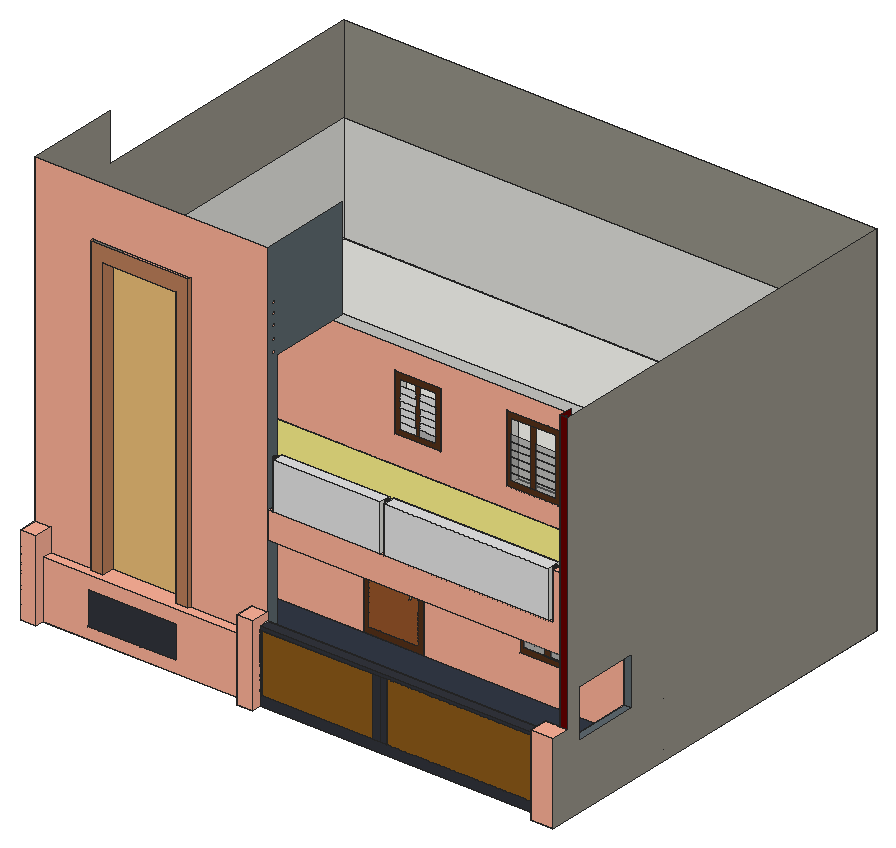
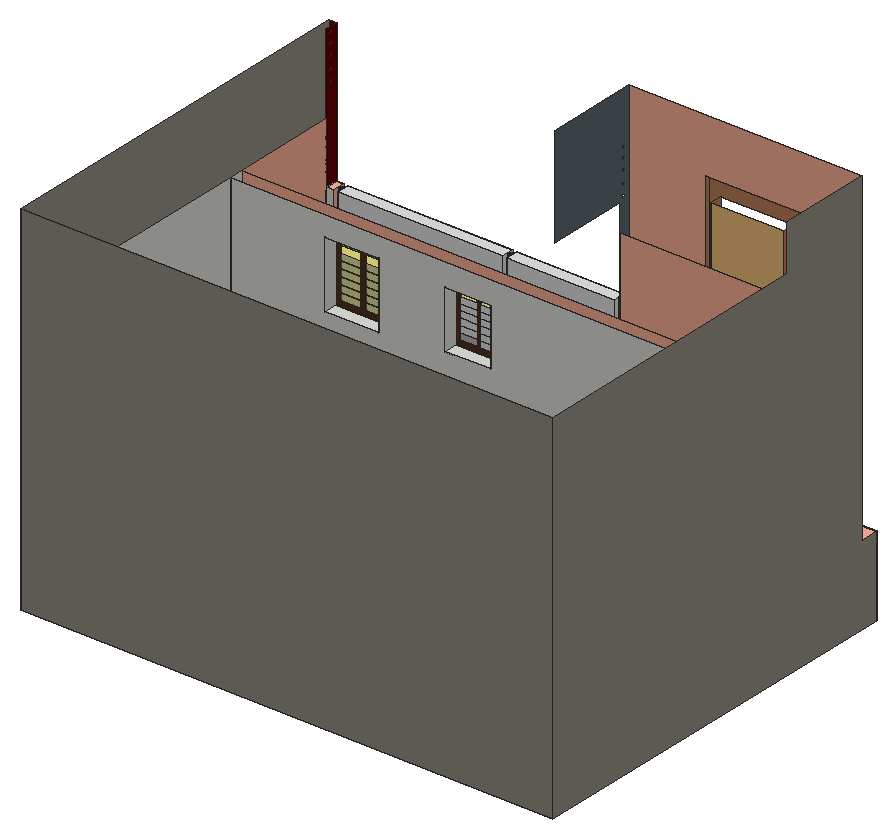
# SketchUp Ruby script. Lengths in inches.
U = 1.inch
M = Sketchup.active_model
def pt(a) = Geom::Point3d.new(a.map { |v| v * U })
def face(e, loops, mat)
  f = e.add_face(loops[0].map { |a| pt(a) })
  loops[1..].each { |l| e.add_face(l.map { |a| pt(a) }).erase! }
  f.material = f.back_material = mat if mat
  f
end
# faces: each face lists its corners as indices into pts; further lists are holes
def faces(e, pts, list, mat = nil) = list.each { |f| face(e, (f[0].is_a?(Array) ? f : [f]).map { |l| l.map { |i| pts[i] } }, mat) }
# xy, xz, yz: faces in a plane at the given z, y or x. An outline is a flat list of corners, or four numbers for a rectangle; further outlines are holes
def ring(l) = l.size == 4 ? [[l[0], l[1]], [l[2], l[1]], [l[2], l[3]], [l[0], l[3]]] : l.each_slice(2).to_a
def flat(e, list, mat, &to3) = list.each { |f| face(e, (f[0].is_a?(Array) ? f : [f]).map { |l| ring(l).map { |u, v| to3.(u, v) } }, mat) }
def xy(e, z, list, mat = nil) = flat(e, list, mat) { |x, y| [x, y, z] }
def xz(e, y, list, mat = nil) = flat(e, list, mat) { |x, z| [x, y, z] }
def yz(e, x, list, mat = nil) = flat(e, list, mat) { |y, z| [x, y, z] }
def lines(e, pts, list) = list.each { |a, b| e.add_line(pt(pts[a]), pt(pts[b])) }
# prism: a flat outline (further loops are holes) pulled along v
def prism(e, loops, v, mat = nil)
  f = face(e, loops, mat); d = Geom::Vector3d.new(v.map { |x| x * U })
  f.pushpull(f.normal.samedirection?(d) ? d.length : -d.length)
end
def box(e, o, s, mat = nil) = prism(e, [[o, [o[0] + s[0], o[1], o[2]], [o[0] + s[0], o[1] + s[1], o[2]], [o[0], o[1] + s[1], o[2]]]], [0, 0, s[2]], mat)
def at(x, y, z, deg = 0) = Geom::Transformation.translation(pt([x, y, z])) * Geom::Transformation.rotation(ORIGIN, Z_AXIS, deg.degrees)
def axes(o, x, y, z) = Geom::Transformation.new([*x, 0, *y, 0, *z, 0, *pt(o).to_a, 1])
def part(name) = M.definitions.add(name)
# library, detail: a bought-in or finely detailed component or shape, given as its bounding box
def library(name, o, s) = part(name).tap { |d| box(d.entities, o, s) }
def detail(e, o, s) = box(e.add_group.entities, o, s)
def put(e, d, t, mat = nil) = e.add_instance(d, t).tap { |i| i.material = mat if mat }
def group(e, t, mat = nil) = e.add_group.tap { |g| g.transformation = t; g.material = mat if mat }.entities
root = M.entities
M.materials.add("[Blinds Weave]").color = [141, 91, 25]
M.materials.add("[Carpet Diamond Yellow]").color = [226, 217, 124]
M.materials.add("[Color A08]").color = [102, 0, 0]
M.materials.add("[Color B02]").color = [255, 178, 153]
M.materials.add("[Formica Graystone]").color = [149, 146, 135]
M.materials.add("[Formica Laminate Dark]").color = [50, 53, 60]
M.materials.add("[Formica Speckled Grey]").color = [94, 105, 111]
M.materials.add("[Mirror 01]").color = [185, 185, 185]
M.materials.add("[Mirror 02]").color = [229, 229, 229]
M.materials.add("[Suede Blue]").color = [50, 57, 70]
M.materials.add("[Translucent Glass Gray]").color = [128, 128, 128]
M.materials["[Translucent Glass Gray]"].alpha = 0.5
M.materials.add("[Wood Cherry Original]").color = [152, 86, 42]
M.materials.add("[Wood Floor Light]").color = [204, 176, 127]
M.materials.add("[Wood OSB]").color = [240, 195, 122]
M.materials.add("[Wood Veneer 01]").color = [84, 49, 25]
M.materials.add("[Wood Veneer 02]").color = [190, 128, 91]
xy(root,0,[[0,0,0,368.0625,485.46,368.0625,485.46,0,464.69,0,464.69,8.0625,211.9,8.0625,211.9,0,197.32,0,197.32,8.0625,14.5,8.0625,14.5,0]])
xy(root,9.18,[[211.9,8.0625,213.81,17.0625],[213.81,8.0625,314.67,17.0625],[314.67,8.0625,327.25,17.0625],[327.25,8.0625,462.45,17.0625],[462.45,8.0625,464.69,17.0625],
  [212.41,125.15,267.59,137.68],[7.28,137.68,478.18,359.0625]])
xy(root,9.18,[[211.9,17.0625,478.18,17.0625,478.18,125.15,7.28,125.15,7.28,27.5,211.9,27.5]],"[Suede Blue]")
xy(root,52.35,[[14.5,8.0625,197.32,8.0625,197.32,17.0625,141.31,17.0625,141.31,14.6875,129.94,14.6875,129.94,25.8125,63.47,25.8125,63.47,14.6875,52.1,14.6875,52.1,17.0625,14.5,17.0625]],"[Color B02]")
xy(root,58.9,[[478.18,28.71,485.46,90.15]],"[Formica Speckled Grey]")
xy(root,62.67,[[213.81,8.0625,314.67,17.0625],[314.67,8.0625,327.25,17.0625],[327.25,8.0625,462.45,17.0625]])
xy(root,65.67,[[211.9,8.0625,464.69,17.0625]],"[Formica Laminate Dark]")
xy(root,73.06,[[0,0,14.5,17.0625],[197.32,0,211.9,17.0625],[464.69,0,485.46,17.0625]],"[Color B02]")
xy(root,102.66,[[478.18,28.71,485.46,90.15]],"[Formica Speckled Grey]")
xy(root,115.45,[[212.41,125.15,267.59,137.68]])
xy(root,131.58,[[7.28,125.15,478.18,137.68],[7.28,137.68,478.18,359.0625]])
xy(root,131.58,[[211.9,17.0625,211.9,27.5,7.28,27.5,7.28,125.15,478.18,125.15,478.18,17.0625]],"[Color B02]")
xy(root,156.06,[[216.17,17.0625,314.19,17.0625,314.19,27.97,216.17,27.53],[317.77,17.0625,467.97,17.0625,467.97,28.67,317.77,27.98],[214.59,20.61,214.22,20.67,213.88,20.85,213.58,21.125,213.36,21.49,213.22,21.91,213.17,22.36,213.22,22.82,213.36,23.24,213.58,23.6,213.88,23.88,214.22,24.05,214.59,24.11,214.95,24.05,215.29,23.88,215.59,23.6,215.8125,23.24,215.95,22.82,216,22.36,215.95,21.91,215.8125,21.49,215.59,21.125,215.29,20.85,214.95,20.67],[316.03,20.61,315.66,20.67,315.32,20.85,315.02,21.125,314.8,21.49,314.66,21.91,314.61,22.36,314.66,22.82,314.8,23.24,315.02,23.6,315.32,23.88,315.66,24.05,316.03,24.11,316.39,24.05,316.73,23.88,317.03,23.6,317.25,23.24,317.39,22.82,317.44,22.36,317.39,21.91,317.25,21.49,317.03,21.125,316.73,20.85,316.39,20.67],[469.7,20.61,469.34,20.67,469,20.85,468.7,21.125,468.48,21.49,468.34,21.91,468.29,22.36,468.34,22.82,468.48,23.24,468.7,23.6,469,23.88,469.34,24.05,469.7,24.11,470.07,24.05,470.41,23.88,470.71,23.6,470.93,23.24,471.07,22.82,471.12,22.36,471.07,21.91,470.93,21.49,470.71,21.125,470.41,20.85,470.07,20.67],
  [7.28,137.68,478.18,359.0625]])
xy(root,156.06,[[7.28,27.5,211.9,27.5,216.17,27.53,314.19,27.97,317.77,27.98,467.97,28.67,471.32,28.68,478.18,28.71,478.18,125.15,7.28,125.15]],"[Carpet Diamond Yellow]")
xy(root,156.06,[[[211.9,17.0625,216.17,17.0625,216.17,27.53,211.9,27.5],[214.59,20.61,214.22,20.67,213.88,20.85,213.58,21.125,213.36,21.49,213.22,21.91,213.17,22.36,213.22,22.82,213.36,23.24,213.58,23.6,213.88,23.88,214.22,24.05,214.59,24.11,214.95,24.05,215.29,23.88,215.59,23.6,215.8125,23.24,215.95,22.82,216,22.36,215.95,21.91,215.8125,21.49,215.59,21.125,215.29,20.85,214.95,20.67]],[[314.19,17.0625,317.77,17.0625,317.77,27.98,314.19,27.97],[316.03,20.61,315.66,20.67,315.32,20.85,315.02,21.125,314.8,21.49,314.66,21.91,314.61,22.36,314.66,22.82,314.8,23.24,315.02,23.6,315.32,23.88,315.66,24.05,316.03,24.11,316.39,24.05,316.73,23.88,317.03,23.6,317.25,23.24,317.39,22.82,317.44,22.36,317.39,21.91,317.25,21.49,317.03,21.125,316.73,20.85,316.39,20.67]],[[467.97,17.0625,471.32,17.0625,471.32,28.68,467.97,28.67],[469.7,20.61,469.34,20.67,469,20.85,468.7,21.125,468.48,21.49,468.34,21.91,468.29,22.36,468.34,22.82,468.48,23.24,468.7,23.6,469,23.88,469.34,24.05,469.7,24.11,470.07,24.05,470.41,23.88,470.71,23.6,470.93,23.24,471.07,22.82,471.12,22.36,471.07,21.91,470.93,21.49,470.71,21.125,470.41,20.85,470.07,20.67]]],"[Color B02]")
xy(root,174.9375,[[343.11,125.15,391.96,137.68]])
xy(root,181.03,[[241.28,125.15,282.74,137.68]])
xy(root,198.52,[[471.32,17.0625,478.18,17.0625,478.18,28.71,471.32,28.68]],"[Color B02]")
xy(root,198.52,[[214.59,20.61,214.95,20.67,215.29,20.85,215.59,21.125,215.8125,21.49,215.95,21.91,216,22.36,215.95,22.82,215.8125,23.24,215.59,23.6,215.29,23.88,214.95,24.05,214.59,24.11,214.22,24.05,213.88,23.88,213.58,23.6,213.36,23.24,213.22,22.82,213.17,22.36,213.22,21.91,213.36,21.49,213.58,21.125,213.88,20.85,214.22,20.67],[316.03,20.61,316.39,20.67,316.73,20.85,317.03,21.125,317.25,21.49,317.39,21.91,317.44,22.36,317.39,22.82,317.25,23.24,317.03,23.6,316.73,23.88,316.39,24.05,316.03,24.11,315.66,24.05,315.32,23.88,315.02,23.6,314.8,23.24,314.66,22.82,314.61,22.36,314.66,21.91,314.8,21.49,315.02,21.125,315.32,20.85,315.66,20.67],[469.7,20.61,470.07,20.67,470.41,20.85,470.71,21.125,470.93,21.49,471.07,21.91,471.12,22.36,471.07,22.82,470.93,23.24,470.71,23.6,470.41,23.88,470.07,24.05,469.7,24.11,469.34,24.05,469,23.88,468.7,23.6,468.48,23.24,468.34,22.82,468.29,22.36,468.34,21.91,468.48,21.49,468.7,21.125,469,20.85,469.34,20.67]],"[Formica Laminate Dark]")
xy(root,198.52,[[216.17,17.0625,314.19,17.0625,314.19,27.97,216.17,27.53],[317.77,17.0625,467.97,17.0625,467.97,28.67,317.77,27.98]],"[Mirror 02]")
xz(root,0,[[0,0,14.5,73.06],[197.32,0,211.9,73.06],[464.69,0,485.46,73.06]],"[Color B02]")
xz(root,8.0625,[[213.81,9.18,314.67,62.67],[327.25,9.18,462.45,62.67]],"[Blinds Weave]")
xz(root,8.0625,[[[14.5,0,197.32,52.35],[55.27,10.18,136.02,40.68]]],"[Color B02]")
xz(root,8.0625,[[211.9,0,464.69,9.18],[211.9,9.18,213.81,62.67],[314.67,9.18,320.96,62.67],[320.96,9.18,327.25,62.67],[462.45,9.18,464.69,62.67],
  [55.27,10.18,136.02,40.68],[211.9,62.67,464.69,65.67]],"[Formica Laminate Dark]")
xz(root,14.6875,[[52.1,52.35,63.47,52.35,63.47,306.94,129.94,306.94,129.94,52.35,141.31,52.35,141.31,321.27,52.1,321.27]],"[Wood Veneer 02]")
xz(root,17.0625,[[464.69,9.18,478.18,73.06]])
xz(root,17.0625,[[213.81,9.18,314.67,62.67],[327.25,9.18,462.45,62.67]],"[Blinds Weave]")
xz(root,17.0625,[[478.18,73.06,485.46,327.42]],"[Color A08]")
xz(root,17.0625,[[14.5,52.35,52.1,52.35,52.1,321.27,141.31,321.27,141.31,52.35,197.32,52.35,197.32,73.06,211.9,73.06,211.9,370.36,0,370.36,0,73.06,14.5,73.06],[211.9,131.58,478.18,131.58,478.18,198.52,471.32,198.52,471.32,156.06,211.9,156.06]],"[Color B02]")
xz(root,17.0625,[[211.9,9.18,213.81,62.67],[314.67,9.18,327.25,62.67],[462.45,9.18,464.69,62.67],[211.9,62.67,464.69,65.67]],"[Formica Laminate Dark]")
xz(root,17.0625,[[216.17,156.06,314.19,198.52],[317.77,156.06,467.97,198.52]],"[Mirror 02]")
xz(root,25.8125,[[63.47,52.35,129.94,306.94]],"[Wood OSB]")
xz(root,27.5,[[7.28,131.58,211.9,156.06]])
xz(root,27.5,[[7.28,9.18,211.9,131.58],[7.28,156.06,211.9,253.98]],"[Color B02]")
xz(root,28.71,[[478.18,58.9,485.46,102.66]],"[Formica Speckled Grey]")
xz(root,90.15,[[478.18,58.9,485.46,102.66]],"[Formica Speckled Grey]")
xz(root,125.15,[[358.66,47.86,377.66,48.07],[377.66,47.86,383.28,48.07],[383.28,47.86,401.9375,48.07],[7.28,131.58,478.18,156.06]])
xz(root,125.15,[[[7.28,9.18,212.41,9.18,212.41,115.45,267.59,115.45,267.59,9.18,478.18,9.18,478.18,131.58,7.28,131.58],[354.59,42.72,406.02,114.1875]],[[7.28,156.06,478.18,253.98],[343.11,174.9375,391.96,236.52],[241.28,181.03,282.74,233.31]]],"[Color B02]")
xz(root,125.15,[[263.78,186.31,278.56,192.2]],"[Mirror 01]")
xz(root,125.15,[[245.46,186.31,260.12,192.2],[245.46,192.2,260.12,198.13],[263.78,192.2,278.56,198.13],[245.46,198.13,260.12,204.0625],[263.78,198.13,278.56,204.0625],
  [245.46,204.0625,260.12,209.99],[263.78,204.0625,278.56,209.99],[245.46,209.99,260.12,215.92],[263.78,209.99,278.56,215.92],[245.46,215.92,260.12,221.85],
  [263.78,215.92,278.56,221.85]],"[Mirror 02]")
xz(root,125.15,[[358.66,48.07,377.66,58.21],[383.28,48.07,401.9375,58.21],[358.66,58.21,377.66,68.35],[383.28,58.21,401.9375,68.35],[358.66,68.35,377.66,78.48],
  [383.28,68.35,401.9375,78.48],[358.66,78.48,377.66,88.62],[383.28,78.48,401.9375,88.62],[358.66,88.62,377.66,98.75],[383.28,88.62,401.9375,98.75],
  [358.66,98.75,377.66,109.05],[383.28,98.75,401.9375,109.05],[346.84,179.64,365.15,186.39],[369.6875,179.64,388.23,186.39],[346.84,186.39,365.15,192.83],
  [369.6875,186.39,388.23,192.83],[346.84,192.83,365.15,199.27],[369.6875,192.83,388.23,199.27],[346.84,199.27,365.15,205.7],[369.6875,199.27,388.23,205.7],
  [346.84,205.7,365.15,212.14],[369.6875,205.7,388.23,212.14],[346.84,212.14,365.15,218.58],[369.6875,212.14,388.23,218.58]],"[Translucent Glass Gray]")
xz(root,125.15,[[[217.68,15.82,262.32,108.81],[253.55,50.5,256.74,74.21]]],"[Wood Cherry Original]")
xz(root,125.15,[[253.55,50.5,256.74,74.21]],"[Wood Floor Light]")
xz(root,125.15,[[[212.41,9.18,267.59,115.45],[217.68,15.82,262.32,108.81]],[[354.59,42.72,406.02,114.1875],[358.66,47.86,401.9375,109.05]],[377.66,48.07,383.28,109.05],[[343.11,174.9375,391.96,236.52],[346.84,179.64,388.23,231.81]],[365.15,179.64,369.6875,231.81],
  [[241.28,181.03,282.74,233.31],[245.46,186.31,278.56,228.03]],[260.12,186.31,263.78,228.03]],"[Wood Veneer 01]")
xz(root,137.68,[[[7.28,9.18,7.28,131.58,478.18,131.58,478.18,9.18,267.59,9.18,267.59,115.45,212.41,115.45,212.41,9.18],[338.76,52.4,367.89,101.36]],[7.28,131.58,478.18,156.06],[[7.28,156.06,478.18,253.98],[343.11,174.9375,391.96,236.52],[241.28,181.03,282.74,233.31]]])
xz(root,359.0625,[[7.28,9.18,478.18,131.58],[7.28,131.58,478.18,156.06],[7.28,156.06,478.18,253.98]])
xz(root,368.0625,[[0,0,485.46,327.42]],"[Formica Graystone]")
yz(root,0,[[0,0,0,73.06,17.0625,73.06,17.0625,370.36,101.5625,370.36,101.5625,327.42,368.0625,327.42,368.0625,0]],"[Formica Graystone]")
yz(root,7.28,[[125.15,9.18,137.68,131.58],[137.68,9.18,359.0625,131.58],[27.5,131.58,125.15,156.06],[125.15,131.58,137.68,253.98],[137.68,131.58,359.0625,156.06],
  [137.68,156.06,359.0625,253.98]])
yz(root,7.28,[[27.5,9.18,125.15,131.58],[27.5,156.06,125.15,253.98]],"[Color B02]")
yz(root,14.5,[[0,0,8.0625,0,8.0625,52.35,17.0625,52.35,17.0625,73.06,0,73.06]],"[Color B02]")
yz(root,52.1,[[14.6875,52.35,17.0625,321.27]],"[Wood Veneer 02]")
yz(root,63.47,[[14.6875,52.35,25.8125,306.94]],"[Wood Veneer 02]")
yz(root,129.94,[[14.6875,52.35,25.8125,306.94]],"[Wood Veneer 02]")
yz(root,141.31,[[14.6875,52.35,17.0625,321.27]],"[Wood Veneer 02]")
yz(root,197.32,[[0,0,0,73.06,17.0625,73.06,17.0625,52.35,8.0625,52.35,8.0625,0]],"[Color B02]")
yz(root,211.9,[[8.0625,9.18,17.0625,62.67],[8.0625,62.67,17.0625,65.67],[17.0625,131.58,27.5,156.06]])
yz(root,211.9,[[0,0,8.0625,0,8.0625,65.67,17.0625,65.67,17.0625,73.06,0,73.06]],"[Color B02]")
yz(root,211.9,[[17.0625,9.18,27.5,131.58],[[17.0625,156.06,27.5,156.06,27.5,278.46,101.5625,278.46,101.5625,370.36,17.0625,370.36],[23.7,280.86,23.25,280.92,22.83,281.1,22.47,281.38,22.1875,281.75,22.01,282.18,21.95,282.64,22.01,283.11,22.1875,283.54,22.47,283.91,22.83,284.19,23.25,284.37,23.7,284.43,24.16,284.37,24.58,284.19,24.94,283.91,25.22,283.54,25.4,283.11,25.45,282.64,25.4,282.18,25.22,281.75,24.94,281.38,24.58,281.1,24.16,280.92],[23.7,321.21,23.25,321.27,22.83,321.45,22.47,321.74,22.1875,322.11,22.01,322.54,21.95,323,22.01,323.46,22.1875,323.89,22.47,324.26,22.83,324.54,23.25,324.72,23.7,324.78,24.16,324.72,24.58,324.54,24.94,324.26,25.22,323.89,25.4,323.46,25.45,323,25.4,322.54,25.22,322.11,24.94,321.74,24.58,321.45,24.16,321.27],[23.7,302.73,23.25,302.79,22.83,302.96,22.47,303.25,22.1875,303.62,22.01,304.05,21.95,304.51,22.01,304.97,22.1875,305.4,22.47,305.77,22.83,306.06,23.25,306.23,23.7,306.3,24.16,306.23,24.58,306.06,24.94,305.77,25.22,305.4,25.4,304.97,25.45,304.51,25.4,304.05,25.22,303.62,24.94,303.25,24.58,302.96,24.16,302.79],[23.7,291,23.25,291.06,22.83,291.23,22.47,291.52,22.1875,291.89,22.01,292.32,21.95,292.78,22.01,293.24,22.1875,293.67,22.47,294.04,22.83,294.33,23.25,294.5,23.7,294.57,24.16,294.5,24.58,294.33,24.94,294.04,25.22,293.67,25.4,293.24,25.45,292.78,25.4,292.32,25.22,291.89,24.94,291.52,24.58,291.23,24.16,291.06],[23.7,312.48,23.25,312.54,22.83,312.72,22.47,313,22.1875,313.37,22.01,313.8,21.95,314.26,22.01,314.73,22.1875,315.16,22.47,315.53,22.83,315.81,23.25,315.99,23.7,316.05,24.16,315.99,24.58,315.81,24.94,315.53,25.22,315.16,25.4,314.73,25.45,314.26,25.4,313.8,25.22,313.37,24.94,313,24.58,312.72,24.16,312.54]]],"[Formica Speckled Grey]")
yz(root,212.41,[[125.15,9.18,137.68,115.45]])
yz(root,213.81,[[8.0625,9.18,17.0625,62.67]])
yz(root,216.17,[[17.0625,156.06,27.53,198.52]])
yz(root,241.28,[[125.15,181.03,137.68,233.31]])
yz(root,267.59,[[125.15,9.18,137.68,115.45]])
yz(root,282.74,[[125.15,181.03,137.68,233.31]])
yz(root,314.19,[[17.0625,156.06,27.97,198.52]])
yz(root,317.77,[[17.0625,156.06,27.98,198.52]])
yz(root,327.25,[[8.0625,9.18,17.0625,62.67]])
yz(root,343.11,[[125.15,174.9375,137.68,236.52]])
yz(root,391.96,[[125.15,174.9375,137.68,236.52]])
yz(root,464.69,[[8.0625,9.18,17.0625,62.67],[8.0625,62.67,17.0625,65.67]])
yz(root,464.69,[[0,0,0,73.06,17.0625,73.06,17.0625,65.67,8.0625,65.67,8.0625,0]],"[Color B02]")
yz(root,467.97,[[17.0625,156.06,28.67,198.52]])
yz(root,471.32,[[17.0625,156.06,28.68,198.52]],"[Color B02]")
yz(root,478.18,[[125.15,9.18,137.68,131.58],[137.68,9.18,359.0625,131.58],[17.0625,131.58,28.71,198.52],[28.71,131.58,125.15,156.06],[125.15,131.58,137.68,253.98],
  [137.68,131.58,359.0625,156.06],[137.68,156.06,359.0625,253.98]])
yz(root,478.18,[[17.0625,9.18,28.71,131.58],[[17.0625,198.52,28.71,327.42],[23.7,280.86,24.16,280.92,24.58,281.1,24.94,281.38,25.22,281.75,25.4,282.18,25.45,282.64,25.4,283.11,25.22,283.54,24.94,283.91,24.58,284.19,24.16,284.37,23.7,284.43,23.25,284.37,22.83,284.19,22.47,283.91,22.1875,283.54,22.01,283.11,21.95,282.64,22.01,282.18,22.1875,281.75,22.47,281.38,22.83,281.1,23.25,280.92],[23.7,321.21,24.16,321.27,24.58,321.45,24.94,321.74,25.22,322.11,25.4,322.54,25.45,323,25.4,323.46,25.22,323.89,24.94,324.26,24.58,324.54,24.16,324.72,23.7,324.78,23.25,324.72,22.83,324.54,22.47,324.26,22.1875,323.89,22.01,323.46,21.95,323,22.01,322.54,22.1875,322.11,22.47,321.74,22.83,321.45,23.25,321.27],[23.7,291,24.16,291.06,24.58,291.23,24.94,291.52,25.22,291.89,25.4,292.32,25.45,292.78,25.4,293.24,25.22,293.67,24.94,294.04,24.58,294.33,24.16,294.5,23.7,294.57,23.25,294.5,22.83,294.33,22.47,294.04,22.1875,293.67,22.01,293.24,21.95,292.78,22.01,292.32,22.1875,291.89,22.47,291.52,22.83,291.23,23.25,291.06],[23.7,302.73,24.16,302.79,24.58,302.96,24.94,303.25,25.22,303.62,25.4,304.05,25.45,304.51,25.4,304.97,25.22,305.4,24.94,305.77,24.58,306.06,24.16,306.23,23.7,306.3,23.25,306.23,22.83,306.06,22.47,305.77,22.1875,305.4,22.01,304.97,21.95,304.51,22.01,304.05,22.1875,303.62,22.47,303.25,22.83,302.96,23.25,302.79],[23.7,312.48,24.16,312.54,24.58,312.72,24.94,313,25.22,313.37,25.4,313.8,25.45,314.26,25.4,314.73,25.22,315.16,24.94,315.53,24.58,315.81,24.16,315.99,23.7,316.05,23.25,315.99,22.83,315.81,22.47,315.53,22.1875,315.16,22.01,314.73,21.95,314.26,22.01,313.8,22.1875,313.37,22.47,313,22.83,312.72,23.25,312.54]]],"[Color A08]")
yz(root,478.18,[[28.71,9.18,28.71,58.9,90.15,58.9,90.15,102.66,28.71,102.66,28.71,131.58,125.15,131.58,125.15,9.18],[28.71,156.06,125.15,253.98]],"[Color B02]")
yz(root,485.46,[[[0,0,368.0625,0,368.0625,327.42,17.0625,327.42,17.0625,73.06,0,73.06],[28.71,58.9,90.15,102.66]]],"[Formica Graystone]")
p = [[214.22,20.67,156.06],[214.59,20.61,156.06],[214.59,20.61,198.52],[214.22,20.67,198.52],[214.95,20.67,156.06],[214.95,20.67,198.52],
  [315.66,20.67,156.06],[316.03,20.61,156.06],[316.03,20.61,198.52],[315.66,20.67,198.52],[316.39,20.67,156.06],[316.39,20.67,198.52],
  [469.34,20.67,156.06],[469.7,20.61,156.06],[469.7,20.61,198.52],[469.34,20.67,198.52],[470.07,20.67,156.06],[470.07,20.67,198.52],
  [213.88,20.85,156.06],[213.88,20.85,198.52],[215.29,20.85,156.06],[215.29,20.85,198.52],[315.32,20.85,156.06],[315.32,20.85,198.52],
  [316.73,20.85,156.06],[316.73,20.85,198.52],[469,20.85,156.06],[469,20.85,198.52],[470.41,20.85,156.06],[470.41,20.85,198.52],
  [213.58,21.125,156.06],[213.58,21.125,198.52],[215.59,21.125,156.06],[215.59,21.125,198.52],[315.02,21.125,156.06],[315.02,21.125,198.52],
  [317.03,21.125,156.06],[317.03,21.125,198.52],[468.7,21.125,156.06],[468.7,21.125,198.52],[470.71,21.125,156.06],[470.71,21.125,198.52],
  [213.36,21.49,156.06],[213.36,21.49,198.52],[215.8125,21.49,156.06],[215.8125,21.49,198.52],[314.8,21.49,156.06],[314.8,21.49,198.52],
  [317.25,21.49,156.06],[317.25,21.49,198.52],[468.48,21.49,156.06],[468.48,21.49,198.52],[470.93,21.49,156.06],[470.93,21.49,198.52],
  [213.22,21.91,156.06],[213.22,21.91,198.52],[215.95,21.91,156.06],[215.95,21.91,198.52],[314.66,21.91,156.06],[314.66,21.91,198.52],
  [317.39,21.91,156.06],[317.39,21.91,198.52],[468.34,21.91,156.06],[468.34,21.91,198.52],[471.07,21.91,156.06],[471.07,21.91,198.52],
  [213.17,22.36,156.06],[213.17,22.36,198.52],[216,22.36,156.06],[216,22.36,198.52],[314.61,22.36,156.06],[314.61,22.36,198.52],
  [317.44,22.36,156.06],[317.44,22.36,198.52],[468.29,22.36,156.06],[468.29,22.36,198.52],[471.12,22.36,156.06],[471.12,22.36,198.52],
  [213.22,22.82,156.06],[213.22,22.82,198.52],[215.95,22.82,156.06],[215.95,22.82,198.52],[314.66,22.82,156.06],[314.66,22.82,198.52],
  [317.39,22.82,156.06],[317.39,22.82,198.52],[468.34,22.82,156.06],[468.34,22.82,198.52],[471.07,22.82,156.06],[471.07,22.82,198.52],
  [213.36,23.24,156.06],[213.36,23.24,198.52],[215.8125,23.24,156.06],[215.8125,23.24,198.52],[314.8,23.24,156.06],[314.8,23.24,198.52],
  [317.25,23.24,156.06],[317.25,23.24,198.52],[468.48,23.24,156.06],[468.48,23.24,198.52],[470.93,23.24,156.06],[470.93,23.24,198.52],
  [213.58,23.6,156.06],[213.58,23.6,198.52],[215.59,23.6,156.06],[215.59,23.6,198.52],[315.02,23.6,156.06],[315.02,23.6,198.52],
  [317.03,23.6,156.06],[317.03,23.6,198.52],[468.7,23.6,156.06],[468.7,23.6,198.52],[470.71,23.6,156.06],[470.71,23.6,198.52],
  [213.88,23.88,156.06],[213.88,23.88,198.52],[215.29,23.88,156.06],[215.29,23.88,198.52],[315.32,23.88,156.06],[315.32,23.88,198.52],
  [316.73,23.88,156.06],[316.73,23.88,198.52],[469,23.88,156.06],[469,23.88,198.52],[470.41,23.88,156.06],[470.41,23.88,198.52],
  [214.22,24.05,156.06],[214.22,24.05,198.52],[214.95,24.05,156.06],[214.95,24.05,198.52],[315.66,24.05,156.06],[315.66,24.05,198.52],
  [316.39,24.05,156.06],[316.39,24.05,198.52],[469.34,24.05,156.06],[469.34,24.05,198.52],[470.07,24.05,156.06],[470.07,24.05,198.52],
  [214.59,24.11,156.06],[214.59,24.11,198.52],[316.03,24.11,156.06],[316.03,24.11,198.52],[469.7,24.11,156.06],[469.7,24.11,198.52],
  [314.19,27.97,156.06],[216.17,27.53,156.06],[216.17,27.53,198.52],[314.19,27.97,198.52],[467.97,28.67,156.06],[317.77,27.98,156.06],
  [317.77,27.98,198.52],[467.97,28.67,198.52],[478.18,28.71,156.06],[471.32,28.68,156.06],[471.32,28.68,198.52],[478.18,28.71,198.52],
  [478.18,125.15,9.18],[485.46,125.15,9.18],[478.18,125.15,51.32],[485.46,125.15,51.32],[338.76,125.15,52.4],[338.76,137.68,52.4],
  [338.76,125.15,101.36],[338.76,137.68,101.36],[367.89,125.15,52.4],[367.89,137.68,52.4],[367.89,125.15,101.36],[367.89,137.68,101.36]]
faces(root,p,[[0,1,2,3],[1,4,5,2],[6,7,8,9],[7,10,11,8],[12,13,14,15],[13,16,17,14],[18,0,3,19],[4,20,21,5],
  [22,6,9,23],[10,24,25,11],[26,12,15,27],[16,28,29,17],[30,18,19,31],[20,32,33,21],[34,22,23,35],[24,36,37,25],
  [38,26,27,39],[28,40,41,29],[42,30,31,43],[32,44,45,33],[46,34,35,47],[36,48,49,37],[50,38,39,51],[40,52,53,41],
  [54,42,43,55],[44,56,57,45],[58,46,47,59],[48,60,61,49],[62,50,51,63],[52,64,65,53],[66,54,55,67],[56,68,69,57],
  [70,58,59,71],[60,72,73,61],[74,62,63,75],[64,76,77,65],[78,66,67,79],[68,80,81,69],[82,70,71,83],[72,84,85,73],
  [86,74,75,87],[76,88,89,77],[90,78,79,91],[80,92,93,81],[94,82,83,95],[84,96,97,85],[98,86,87,99],[88,100,101,89],
  [102,90,91,103],[92,104,105,93],[106,94,95,107],[96,108,109,97],[110,98,99,111],[100,112,113,101],[114,102,103,115],[104,116,117,105],
  [118,106,107,119],[108,120,121,109],[122,110,111,123],[112,124,125,113],[126,114,115,127],[116,128,129,117],[130,118,119,131],[120,132,133,121],
  [134,122,123,135],[124,136,137,125],[138,126,127,139],[128,138,139,129],[140,130,131,141],[132,140,141,133],[142,134,135,143],[136,142,143,137]],"[Formica Laminate Dark]")
faces(root,p,[[144,145,146,147],[148,149,150,151]],"[Mirror 02]")
faces(root,p,[[152,153,154,155]])
lines(root,p,[[156,157],[158,159],[160,161],[162,163],[164,165],[166,167]])
